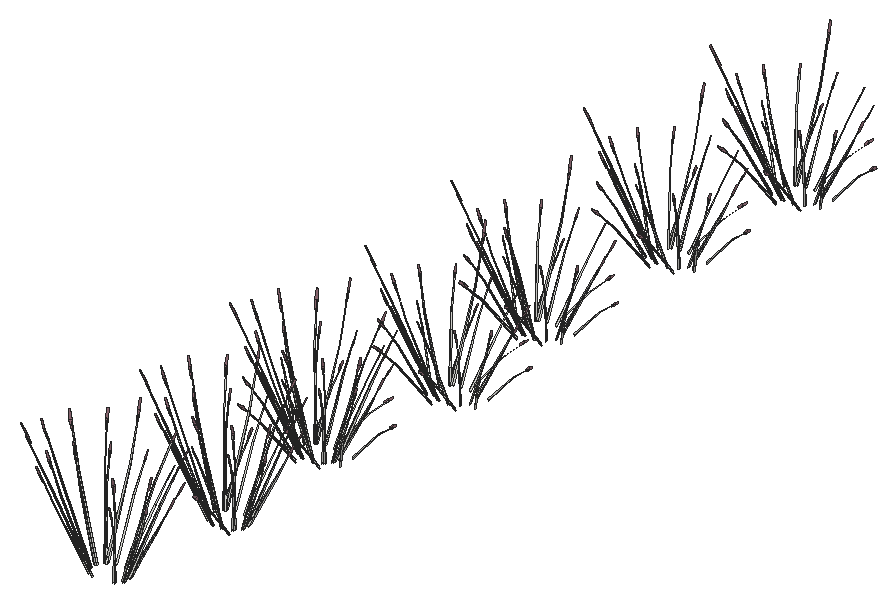
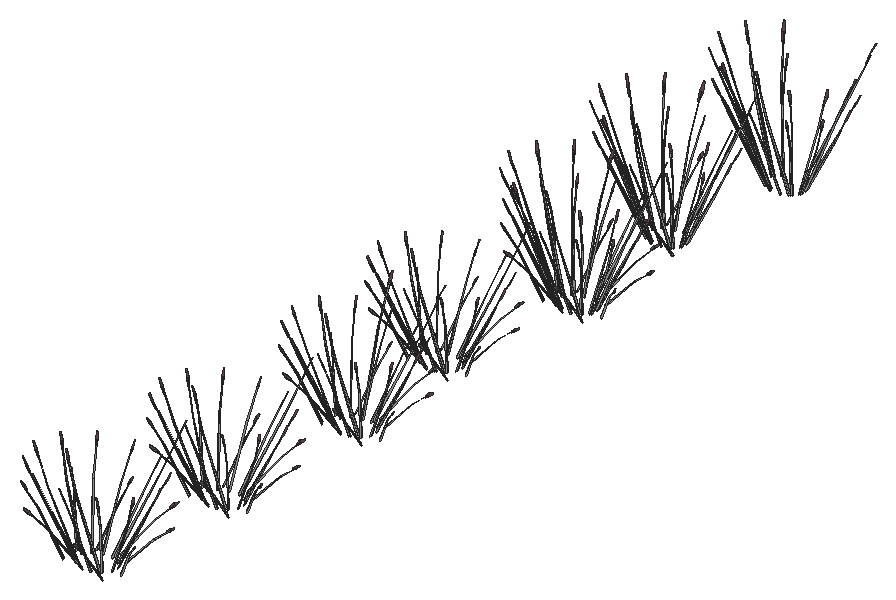
# SketchUp Ruby script. Lengths in inches.
U = 1.inch
M = Sketchup.active_model
def pt(a) = Geom::Point3d.new(a.map { |v| v * U })
def face(e, loops, mat)
  f = e.add_face(loops[0].map { |a| pt(a) })
  loops[1..].each { |l| e.add_face(l.map { |a| pt(a) }).erase! }
  f.material = f.back_material = mat if mat
  f
end
# faces: each face lists its corners as indices into pts; further lists are holes
def faces(e, pts, list, mat = nil) = list.each { |f| face(e, (f[0].is_a?(Array) ? f : [f]).map { |l| l.map { |i| pts[i] } }, mat) }
# xy, xz, yz: faces in a plane at the given z, y or x. An outline is a flat list of corners, or four numbers for a rectangle; further outlines are holes
def ring(l) = l.size == 4 ? [[l[0], l[1]], [l[2], l[1]], [l[2], l[3]], [l[0], l[3]]] : l.each_slice(2).to_a
def flat(e, list, mat, &to3) = list.each { |f| face(e, (f[0].is_a?(Array) ? f : [f]).map { |l| ring(l).map { |u, v| to3.(u, v) } }, mat) }
def xy(e, z, list, mat = nil) = flat(e, list, mat) { |x, y| [x, y, z] }
def xz(e, y, list, mat = nil) = flat(e, list, mat) { |x, z| [x, y, z] }
def yz(e, x, list, mat = nil) = flat(e, list, mat) { |y, z| [x, y, z] }
def lines(e, pts, list) = list.each { |a, b| e.add_line(pt(pts[a]), pt(pts[b])) }
# prism: a flat outline (further loops are holes) pulled along v
def prism(e, loops, v, mat = nil)
  f = face(e, loops, mat); d = Geom::Vector3d.new(v.map { |x| x * U })
  f.pushpull(f.normal.samedirection?(d) ? d.length : -d.length)
end
def box(e, o, s, mat = nil) = prism(e, [[o, [o[0] + s[0], o[1], o[2]], [o[0] + s[0], o[1] + s[1], o[2]], [o[0], o[1] + s[1], o[2]]]], [0, 0, s[2]], mat)
def at(x, y, z, deg = 0) = Geom::Transformation.translation(pt([x, y, z])) * Geom::Transformation.rotation(ORIGIN, Z_AXIS, deg.degrees)
def axes(o, x, y, z) = Geom::Transformation.new([*x, 0, *y, 0, *z, 0, *pt(o).to_a, 1])
def part(name) = M.definitions.add(name)
# library, detail: a bought-in or finely detailed component or shape, given as its bounding box
def library(name, o, s) = part(name).tap { |d| box(d.entities, o, s) }
def detail(e, o, s) = box(e.add_group.entities, o, s)
def put(e, d, t, mat = nil) = e.add_instance(d, t).tap { |i| i.material = mat if mat }
def group(e, t, mat = nil) = e.add_group.tap { |g| g.transformation = t; g.material = mat if mat }.entities
root = M.entities
M.materials.add("LightPink_Translucent").color = [144, 107, 117]
c1 = part("blade")
p = [[2.15,0.21,22],[0,0.17,0],[0.09,0.45,0],[2.18,0.31,22],[2.29,0.31,22],[0.38,0.45,0],
  [2.48,0.24,33],[2.49,0.24,33],[2.48,0.22,33]]
faces(c1.entities,p,[[0,1,2,3],[4,5,2,3],[6,3,4,7],[8,0,3,6]])
c2 = part("seeds")
p = [[0.3,-0.1,1.38],[-0.01,-0.03,1.59],[-0.01,-0.03,0.03],[0.14,-0.07,-0.07],[0.29,-0.03,3],[0.15,0.01,3.11]]
faces(c2.entities,p,[[0,1,2,3],[1,0,4,5]],"LightPink_Translucent")
c3 = part("blade with seeds")
put(c3.entities,c1,at(0,0,0))
put(c3.entities,c2,axes([2.4,0.25,30.99],[1.5799,-0.05474,1.17369],[-0.12525,1.92788,0.29478],[-0.07173,-0.02425,1.56792]))
put(root,c3,axes([46.34,429.16,46.73],[0.87265,0.70663,0.48003],[-0.92674,0.60943,0.3958],[0.16097,-0.33153,0.9933]))
put(root,c3,axes([41.07,428.13,47.43],[-0.81789,0.99285,-0.13619],[-1.18445,-0.572,-0.75594],[-0.41173,-0.28051,1.14864]))
put(root,c3,axes([46.66,429.23,46.73],[1.00708,0.04826,0.0643],[-0.02761,0.72867,0.50621],[0.10538,-0.27912,0.77189]))
put(root,c3,axes([38.21,429.49,46.73],[0.06171,-0.78753,0.0643],[0.9318,0.02159,0.50621],[-0.35694,-0.08241,0.77189]))
put(root,c3,axes([48.3125,431.27,46.73],[0.8413,0.43556,0.0643],[-0.48981,0.62025,0.50621],[0.26973,-0.20053,0.77189]))
put(root,c3,axes([48.08,431.09,46.73],[0.30393,0.95317,0.48003],[-1.19224,0.16542,0.3958],[0.35138,-0.22417,0.9933]))
put(root,c3,axes([36.85,431.89,46.73],[0.34623,-0.9443,0.48003],[1.13828,0.3229,0.3958],[-0.44763,0.05675,0.9933]))
put(root,c3,axes([36.77,431.64,46.73],[-0.4501,-0.70615,0.0643],[0.82077,-0.34564,0.50621],[-0.36181,0.0682,0.77189]))
put(root,c3,axes([48.4375,433.69,46.73],[0.4501,0.70615,0.0643],[-0.82077,0.34564,0.50621],[0.36181,-0.0682,0.77189]))
put(root,c3,axes([48.35,433.44,46.73],[-0.34623,0.9443,0.48003],[-1.13828,-0.3229,0.3958],[0.44763,-0.05675,0.9933]))
put(root,c3,axes([37.13,434.24,46.73],[-0.30393,-0.95317,0.48003],[1.19224,-0.16542,0.3958],[-0.35138,0.22417,0.9933]))
put(root,c3,axes([36.89,434.06,46.73],[-0.8413,-0.43556,0.0643],[0.48981,-0.62025,0.50621],[-0.26973,0.20053,0.77189]))
put(root,c3,axes([47,435.84,46.73],[-0.06171,0.78753,0.0643],[-0.9318,-0.02159,0.50621],[0.35694,0.08241,0.77189]))
put(root,c3,axes([47.09,435.58,46.73],[-0.90362,0.68241,0.48003],[-0.77932,-0.72471,0.3958],[0.42395,0.12588,0.9933]))
put(root,c3,axes([38.55,436.1,46.73],[-1.00708,-0.04826,0.0643],[0.02761,-0.72867,0.50621],[-0.10538,0.27912,0.77189]))
put(root,c3,axes([38.87,436.17,46.73],[-0.87265,-0.70663,0.48003],[0.92674,-0.60943,0.3958],[-0.16097,0.33153,0.9933]))
put(root,c3,axes([44.38,437.13,46.73],[-0.55698,0.6579,0.0643],[-0.79316,-0.38303,0.50621],[0.25643,0.21093,0.77189]))
put(root,c3,axes([44.62,436.95,46.73],[-1.21888,0.23767,0.48003],[-0.21154,-0.93233,0.3958],[0.28666,0.27478,0.9933]))
put(root,c3,axes([41.29,437.23,46.73],[-0.90301,0.35198,0.0643],[-0.44199,-0.64184,0.50621],[0.08721,0.28293,0.77189]))
put(root,c3,axes([38.77,435.76,47.4],[1.34686,0.05131,-0.13498],[-0.03681,0.97156,-0.74919],[-0.09356,0.37418,1.13838]))
put(root,c3,axes([53.75,466.55,46.71],[-0.12446,0.07911,1.77383],[-1.21937,-0.26689,-0.16761],[-0.04414,-0.34521,0.31391]))
put(root,c3,axes([49.95,467.43,46.73],[1.20755,0.27075,0.48003],[-0.41292,0.89013,0.3958],[-0.07257,-0.35005,0.9933]))
put(root,c3,axes([50.27,467.37,46.73],[0.90301,-0.35198,0.0643],[0.44199,0.64184,0.50621],[-0.08721,-0.28293,0.77189]))
put(root,c3,axes([47.18,467.46,46.73],[0.55698,-0.6579,0.0643],[0.79316,0.38303,0.50621],[-0.25643,-0.21093,0.77189]))
put(root,c3,axes([52.69,468.42,46.73],[0.87265,0.70663,0.48003],[-0.92674,0.60943,0.3958],[0.16097,-0.33153,0.9933]))
put(root,c3,axes([47.43,467.4,47.43],[-0.81789,0.99285,-0.13619],[-1.18445,-0.572,-0.75594],[-0.41173,-0.28051,1.14864]))
put(root,c3,axes([53.01,468.49,46.73],[1.00708,0.04826,0.0643],[-0.02761,0.72867,0.50621],[0.10538,-0.27912,0.77189]))
put(root,c3,axes([44.5625,468.76,46.73],[0.06171,-0.78753,0.0643],[0.9318,0.02159,0.50621],[-0.35694,-0.08241,0.77189]))
put(root,c3,axes([54.67,470.54,46.73],[0.8413,0.43556,0.0643],[-0.48981,0.62025,0.50621],[0.26973,-0.20053,0.77189]))
put(root,c3,axes([54.43,470.35,46.73],[0.30393,0.95317,0.48003],[-1.19224,0.16542,0.3958],[0.35138,-0.22417,0.9933]))
put(root,c3,axes([43.21,471.15,46.73],[0.34623,-0.9443,0.48003],[1.13828,0.3229,0.3958],[-0.44763,0.05675,0.9933]))
put(root,c3,axes([43.12,470.9,46.73],[-0.4501,-0.70615,0.0643],[0.82077,-0.34564,0.50621],[-0.36181,0.0682,0.77189]))
put(root,c3,axes([54.79,472.96,46.73],[0.4501,0.70615,0.0643],[-0.82077,0.34564,0.50621],[0.36181,-0.0682,0.77189]))
put(root,c3,axes([54.71,472.71,46.73],[-0.34623,0.9443,0.48003],[-1.13828,-0.3229,0.3958],[0.44763,-0.05675,0.9933]))
put(root,c3,axes([43.48,473.51,46.73],[-0.30393,-0.95317,0.48003],[1.19224,-0.16542,0.3958],[-0.35138,0.22417,0.9933]))
put(root,c3,axes([43.25,473.32,46.73],[-0.8413,-0.43556,0.0643],[0.48981,-0.62025,0.50621],[-0.26973,0.20053,0.77189]))
put(root,c3,axes([53.36,475.1,46.73],[-0.06171,0.78753,0.0643],[-0.9318,-0.02159,0.50621],[0.35694,0.08241,0.77189]))
put(root,c3,axes([53.44,474.85,46.73],[-0.90362,0.68241,0.48003],[-0.77932,-0.72471,0.3958],[0.42395,0.12588,0.9933]))
put(root,c3,axes([44.9,475.37,46.73],[-1.00708,-0.04826,0.0643],[0.02761,-0.72867,0.50621],[-0.10538,0.27912,0.77189]))
put(root,c3,axes([45.23,475.4375,46.73],[-0.87265,-0.70663,0.48003],[0.92674,-0.60943,0.3958],[-0.16097,0.33153,0.9933]))
put(root,c3,axes([50.74,476.4,46.73],[-0.55698,0.6579,0.0643],[-0.79316,-0.38303,0.50621],[0.25643,0.21093,0.77189]))
put(root,c3,axes([50.97,476.21,46.73],[-1.21888,0.23767,0.48003],[-0.21154,-0.93233,0.3958],[0.28666,0.27478,0.9933]))
put(root,c3,axes([47.65,476.49,46.73],[-0.90301,0.35198,0.0643],[-0.44199,-0.64184,0.50621],[0.08721,0.28293,0.77189]))
put(root,c3,axes([45.13,475.02,47.4],[1.34686,0.05131,-0.13498],[-0.03681,0.97156,-0.74919],[-0.09356,0.37418,1.13838]))
put(root,c3,axes([42.27,477.59,46.71],[0.13903,-0.06253,1.77383],[1.14912,0.41591,-0.16761],[-0.027,0.34629,0.31391]))
put(root,c3,axes([50.13,506.81,46.71],[-0.12446,0.07911,1.77383],[-1.21937,-0.26689,-0.16761],[-0.04414,-0.34521,0.31391]))
put(root,c3,axes([43.5,505.29,46.71],[-0.02286,0.12414,1.77383],[-1.12758,0.45052,-0.16761],[-0.33182,-0.23029,0.31391]))
put(root,c3,axes([46.34,507.69,46.73],[1.20755,0.27075,0.48003],[-0.41292,0.89013,0.3958],[-0.07257,-0.35005,0.9933]))
put(root,c3,axes([46.66,507.625,46.73],[0.90301,-0.35198,0.0643],[0.44199,0.64184,0.50621],[-0.08721,-0.28293,0.77189]))
put(root,c3,axes([43.5625,507.72,46.73],[0.55698,-0.6579,0.0643],[0.79316,0.38303,0.50621],[-0.25643,-0.21093,0.77189]))
put(root,c3,axes([49.08,508.68,46.73],[0.87265,0.70663,0.48003],[-0.92674,0.60943,0.3958],[0.16097,-0.33153,0.9933]))
put(root,c3,axes([43.8125,507.65,47.43],[-0.81789,0.99285,-0.13619],[-1.18445,-0.572,-0.75594],[-0.41173,-0.28051,1.14864]))
put(root,c3,axes([49.4,508.75,46.73],[1.00708,0.04826,0.0643],[-0.02761,0.72867,0.50621],[0.10538,-0.27912,0.77189]))
put(root,c3,axes([53.43,510.76,46.71],[-0.16006,-0.00787,1.77383],[-0.66468,-0.8428,-0.16761],[0.26693,-0.27711,0.31391]))
put(root,c3,axes([40.95,509.02,46.73],[0.06171,-0.78753,0.0643],[0.9318,0.02159,0.50621],[-0.35694,-0.08241,0.77189]))
put(root,c3,axes([51.05,510.8,46.73],[0.8413,0.43556,0.0643],[-0.48981,0.62025,0.50621],[0.26973,-0.20053,0.77189]))
put(root,c3,axes([50.82,510.61,46.73],[0.30393,0.95317,0.48003],[-1.19224,0.16542,0.3958],[0.35138,-0.22417,0.9933]))
put(root,c3,axes([39.66,507.99,46.71],[0.09085,0.10335,1.77383],[-0.43798,0.92907,-0.16761],[-0.44357,0.00672,0.31391]))
put(root,c3,axes([39.59,511.41,46.73],[0.34623,-0.9443,0.48003],[1.13828,0.3229,0.3958],[-0.44763,0.05675,0.9933]))
put(root,c3,axes([39.51,511.16,46.73],[-0.4501,-0.70615,0.0643],[0.82077,-0.34564,0.50621],[-0.36181,0.0682,0.77189]))
put(root,c3,axes([51.18,513.21,46.73],[0.4501,0.70615,0.0643],[-0.82077,0.34564,0.50621],[0.36181,-0.0682,0.77189]))
put(root,c3,axes([51.09,512.96,46.73],[-0.34623,0.9443,0.48003],[-1.13828,-0.3229,0.3958],[0.44763,-0.05675,0.9933]))
put(root,c3,axes([53.14,516.02,46.71],[-0.11081,-0.09067,1.77383],[0.2424,-0.97188,-0.16761],[0.43649,-0.06209,0.31391]))
put(root,c3,axes([39.87,513.76,46.73],[-0.30393,-0.95317,0.48003],[1.19224,-0.16542,0.3958],[-0.35138,0.22417,0.9933]))
put(root,c3,axes([39.63,513.58,46.73],[-0.8413,-0.43556,0.0643],[0.48981,-0.62025,0.50621],[-0.26973,0.20053,0.77189]))
put(root,c3,axes([36.49,513.07,46.71],[0.1564,0.02778,1.77383],[0.48382,0.91506,-0.16761],[-0.32016,0.24017,0.31391]))
put(root,c3,axes([49.74,515.36,46.73],[-0.06171,0.78753,0.0643],[-0.9318,-0.02159,0.50621],[0.35694,0.08241,0.77189]))
put(root,c3,axes([49.83,515.11,46.73],[-0.90362,0.68241,0.48003],[-0.77932,-0.72471,0.3958],[0.42395,0.12588,0.9933]))
put(root,c3,axes([45.9,517.07,46.71],[0.00363,-0.12539,1.77383],[1.0502,-0.55319,-0.16761],[0.36479,0.19745,0.31391]))
put(root,c3,axes([41.29,515.63,46.73],[-1.00708,-0.04826,0.0643],[0.02761,-0.72867,0.50621],[-0.10538,0.27912,0.77189]))
put(root,c3,axes([41.61,515.69,46.73],[-0.87265,-0.70663,0.48003],[0.92674,-0.60943,0.3958],[-0.16097,0.33153,0.9933]))
put(root,c3,axes([47.125,516.65,46.73],[-0.55698,0.6579,0.0643],[-0.79316,-0.38303,0.50621],[0.25643,0.21093,0.77189]))
put(root,c3,axes([47.36,516.47,46.73],[-1.21888,0.23767,0.48003],[-0.21154,-0.93233,0.3958],[0.28666,0.27478,0.9933]))
put(root,c3,axes([44.03,516.75,46.73],[-0.90301,0.35198,0.0643],[-0.44199,-0.64184,0.50621],[0.08721,0.28293,0.77189]))
put(root,c3,axes([41.51,515.28,47.4],[1.34686,0.05131,-0.13498],[-0.03681,0.97156,-0.74919],[-0.09356,0.37418,1.13838]))
put(root,c3,axes([38.65,517.85,46.71],[0.13903,-0.06253,1.77383],[1.14912,0.41591,-0.16761],[-0.027,0.34629,0.31391]))
put(root,c3,axes([58.1,550.49,46.71],[-0.12446,0.07911,1.77383],[-1.21937,-0.26689,-0.16761],[-0.04414,-0.34521,0.31391]))
put(root,c3,axes([51.46,548.97,46.71],[-0.02286,0.12414,1.77383],[-1.12758,0.45052,-0.16761],[-0.33182,-0.23029,0.31391]))
put(root,c3,axes([54.625,551.3,46.73],[0.90301,-0.35198,0.0643],[0.44199,0.64184,0.50621],[-0.08721,-0.28293,0.77189]))
put(root,c3,axes([51.53,551.4,46.73],[0.55698,-0.6579,0.0643],[0.79316,0.38303,0.50621],[-0.25643,-0.21093,0.77189]))
put(root,c3,axes([51.78,551.33,47.43],[-0.81789,0.99285,-0.13619],[-1.18445,-0.572,-0.75594],[-0.41173,-0.28051,1.14864]))
put(root,c3,axes([57.37,552.42,46.73],[1.00708,0.04826,0.0643],[-0.02761,0.72867,0.50621],[0.10538,-0.27912,0.77189]))
put(root,c3,axes([61.4,554.43,46.71],[-0.16006,-0.00787,1.77383],[-0.66468,-0.8428,-0.16761],[0.26693,-0.27711,0.31391]))
put(root,c3,axes([48.91,552.69,46.73],[0.06171,-0.78753,0.0643],[0.9318,0.02159,0.50621],[-0.35694,-0.08241,0.77189]))
put(root,c3,axes([59.02,554.47,46.73],[0.8413,0.43556,0.0643],[-0.48981,0.62025,0.50621],[0.26973,-0.20053,0.77189]))
put(root,c3,axes([47.63,551.66,46.71],[0.09085,0.10335,1.77383],[-0.43798,0.92907,-0.16761],[-0.44357,0.00672,0.31391]))
put(root,c3,axes([47.48,554.84,46.73],[-0.4501,-0.70615,0.0643],[0.82077,-0.34564,0.50621],[-0.36181,0.0682,0.77189]))
put(root,c3,axes([59.15,556.89,46.73],[0.4501,0.70615,0.0643],[-0.82077,0.34564,0.50621],[0.36181,-0.0682,0.77189]))
put(root,c3,axes([61.11,559.7,46.71],[-0.11081,-0.09067,1.77383],[0.2424,-0.97188,-0.16761],[0.43649,-0.06209,0.31391]))
put(root,c3,axes([47.6,557.26,46.73],[-0.8413,-0.43556,0.0643],[0.48981,-0.62025,0.50621],[-0.26973,0.20053,0.77189]))
put(root,c3,axes([44.46,556.75,46.71],[0.1564,0.02778,1.77383],[0.48382,0.91506,-0.16761],[-0.32016,0.24017,0.31391]))
put(root,c3,axes([57.71,559.03,46.73],[-0.06171,0.78753,0.0643],[-0.9318,-0.02159,0.50621],[0.35694,0.08241,0.77189]))
put(root,c3,axes([53.87,560.74,46.71],[0.00363,-0.12539,1.77383],[1.0502,-0.55319,-0.16761],[0.36479,0.19745,0.31391]))
put(root,c3,axes([49.26,559.3,46.73],[-1.00708,-0.04826,0.0643],[0.02761,-0.72867,0.50621],[-0.10538,0.27912,0.77189]))
put(root,c3,axes([55.09,560.33,46.73],[-0.55698,0.6579,0.0643],[-0.79316,-0.38303,0.50621],[0.25643,0.21093,0.77189]))
put(root,c3,axes([52,560.43,46.73],[-0.90301,0.35198,0.0643],[-0.44199,-0.64184,0.50621],[0.08721,0.28293,0.77189]))
put(root,c3,axes([49.48,558.96,47.4],[1.34686,0.05131,-0.13498],[-0.03681,0.97156,-0.74919],[-0.09356,0.37418,1.13838]))
put(root,c3,axes([46.62,561.52,46.71],[0.13903,-0.06253,1.77383],[1.14912,0.41591,-0.16761],[-0.027,0.34629,0.31391]))
put(root,c3,axes([54.27,589.3125,46.71],[-0.12446,0.07911,1.77383],[-1.21937,-0.26689,-0.16761],[-0.04414,-0.34521,0.31391]))
put(root,c3,axes([47.63,587.79,46.71],[-0.02286,0.12414,1.77383],[-1.12758,0.45052,-0.16761],[-0.33182,-0.23029,0.31391]))
put(root,c3,axes([50.47,590.19,46.73],[1.20755,0.27075,0.48003],[-0.41292,0.89013,0.3958],[-0.07257,-0.35005,0.9933]))
put(root,c3,axes([50.79,590.125,46.73],[0.90301,-0.35198,0.0643],[0.44199,0.64184,0.50621],[-0.08721,-0.28293,0.77189]))
put(root,c3,axes([47.7,590.22,46.73],[0.55698,-0.6579,0.0643],[0.79316,0.38303,0.50621],[-0.25643,-0.21093,0.77189]))
put(root,c3,axes([47.95,590.15,47.43],[-0.81789,0.99285,-0.13619],[-1.18445,-0.572,-0.75594],[-0.41173,-0.28051,1.14864]))
put(root,c3,axes([53.54,591.25,46.73],[1.00708,0.04826,0.0643],[-0.02761,0.72867,0.50621],[0.10538,-0.27912,0.77189]))
put(root,c3,axes([57.57,593.26,46.71],[-0.16006,-0.00787,1.77383],[-0.66468,-0.8428,-0.16761],[0.26693,-0.27711,0.31391]))
put(root,c3,axes([45.08,591.52,46.73],[0.06171,-0.78753,0.0643],[0.9318,0.02159,0.50621],[-0.35694,-0.08241,0.77189]))
put(root,c3,axes([55.19,593.3,46.73],[0.8413,0.43556,0.0643],[-0.48981,0.62025,0.50621],[0.26973,-0.20053,0.77189]))
put(root,c3,axes([43.8,590.49,46.71],[0.09085,0.10335,1.77383],[-0.43798,0.92907,-0.16761],[-0.44357,0.00672,0.31391]))
put(root,c3,axes([43.65,593.66,46.73],[-0.4501,-0.70615,0.0643],[0.82077,-0.34564,0.50621],[-0.36181,0.0682,0.77189]))
put(root,c3,axes([55.32,595.72,46.73],[0.4501,0.70615,0.0643],[-0.82077,0.34564,0.50621],[0.36181,-0.0682,0.77189]))
put(root,c3,axes([57.28,598.52,46.71],[-0.11081,-0.09067,1.77383],[0.2424,-0.97188,-0.16761],[0.43649,-0.06209,0.31391]))
put(root,c3,axes([43.77,596.08,46.73],[-0.8413,-0.43556,0.0643],[0.48981,-0.62025,0.50621],[-0.26973,0.20053,0.77189]))
put(root,c3,axes([40.63,595.57,46.71],[0.1564,0.02778,1.77383],[0.48382,0.91506,-0.16761],[-0.32016,0.24017,0.31391]))
put(root,c3,axes([53.88,597.86,46.73],[-0.06171,0.78753,0.0643],[-0.9318,-0.02159,0.50621],[0.35694,0.08241,0.77189]))
put(root,c3,axes([50.04,599.57,46.71],[0.00363,-0.12539,1.77383],[1.0502,-0.55319,-0.16761],[0.36479,0.19745,0.31391]))
put(root,c3,axes([45.43,598.13,46.73],[-1.00708,-0.04826,0.0643],[0.02761,-0.72867,0.50621],[-0.10538,0.27912,0.77189]))
put(root,c3,axes([51.26,599.15,46.73],[-0.55698,0.6579,0.0643],[-0.79316,-0.38303,0.50621],[0.25643,0.21093,0.77189]))
put(root,c3,axes([48.17,599.25,46.73],[-0.90301,0.35198,0.0643],[-0.44199,-0.64184,0.50621],[0.08721,0.28293,0.77189]))
put(root,c3,axes([45.65,597.78,47.4],[1.34686,0.05131,-0.13498],[-0.03681,0.97156,-0.74919],[-0.09356,0.37418,1.13838]))
put(root,c3,axes([42.79,600.35,46.71],[0.13903,-0.06253,1.77383],[1.14912,0.41591,-0.16761],[-0.027,0.34629,0.31391]))
put(root,c3,axes([57.0625,638.32,46.71],[-0.12446,0.07911,1.77383],[-1.21937,-0.26689,-0.16761],[-0.04414,-0.34521,0.31391]))
put(root,c3,axes([50.43,636.8,46.71],[-0.02286,0.12414,1.77383],[-1.12758,0.45052,-0.16761],[-0.33182,-0.23029,0.31391]))
put(root,c3,axes([53.59,639.14,46.73],[0.90301,-0.35198,0.0643],[0.44199,0.64184,0.50621],[-0.08721,-0.28293,0.77189]))
put(root,c3,axes([50.49,639.23,46.73],[0.55698,-0.6579,0.0643],[0.79316,0.38303,0.50621],[-0.25643,-0.21093,0.77189]))
put(root,c3,axes([50.74,639.16,47.43],[-0.81789,0.99285,-0.13619],[-1.18445,-0.572,-0.75594],[-0.41173,-0.28051,1.14864]))
put(root,c3,axes([56.33,640.26,46.73],[1.00708,0.04826,0.0643],[-0.02761,0.72867,0.50621],[0.10538,-0.27912,0.77189]))
put(root,c3,axes([60.36,642.27,46.71],[-0.16006,-0.00787,1.77383],[-0.66468,-0.8428,-0.16761],[0.26693,-0.27711,0.31391]))
put(root,c3,axes([47.875,640.53,46.73],[0.06171,-0.78753,0.0643],[0.9318,0.02159,0.50621],[-0.35694,-0.08241,0.77189]))
put(root,c3,axes([57.98,642.31,46.73],[0.8413,0.43556,0.0643],[-0.48981,0.62025,0.50621],[0.26973,-0.20053,0.77189]))
put(root,c3,axes([46.59,639.5,46.71],[0.09085,0.10335,1.77383],[-0.43798,0.92907,-0.16761],[-0.44357,0.00672,0.31391]))
put(root,c3,axes([46.4375,642.67,46.73],[-0.4501,-0.70615,0.0643],[0.82077,-0.34564,0.50621],[-0.36181,0.0682,0.77189]))
put(root,c3,axes([58.11,644.72,46.73],[0.4501,0.70615,0.0643],[-0.82077,0.34564,0.50621],[0.36181,-0.0682,0.77189]))
put(root,c3,axes([60.07,647.53,46.71],[-0.11081,-0.09067,1.77383],[0.2424,-0.97188,-0.16761],[0.43649,-0.06209,0.31391]))
put(root,c3,axes([46.5625,645.09,46.73],[-0.8413,-0.43556,0.0643],[0.48981,-0.62025,0.50621],[-0.26973,0.20053,0.77189]))
put(root,c3,axes([43.42,644.58,46.71],[0.1564,0.02778,1.77383],[0.48382,0.91506,-0.16761],[-0.32016,0.24017,0.31391]))
put(root,c3,axes([56.67,646.87,46.73],[-0.06171,0.78753,0.0643],[-0.9318,-0.02159,0.50621],[0.35694,0.08241,0.77189]))
put(root,c3,axes([52.83,648.58,46.71],[0.00363,-0.12539,1.77383],[1.0502,-0.55319,-0.16761],[0.36479,0.19745,0.31391]))
put(root,c3,axes([48.22,647.14,46.73],[-1.00708,-0.04826,0.0643],[0.02761,-0.72867,0.50621],[-0.10538,0.27912,0.77189]))
put(root,c3,axes([54.05,648.16,46.73],[-0.55698,0.6579,0.0643],[-0.79316,-0.38303,0.50621],[0.25643,0.21093,0.77189]))
put(root,c3,axes([50.96,648.26,46.73],[-0.90301,0.35198,0.0643],[-0.44199,-0.64184,0.50621],[0.08721,0.28293,0.77189]))
put(root,c3,axes([48.44,646.79,47.4],[1.34686,0.05131,-0.13498],[-0.03681,0.97156,-0.74919],[-0.09356,0.37418,1.13838]))
put(root,c3,axes([45.58,649.36,46.71],[0.13903,-0.06253,1.77383],[1.14912,0.41591,-0.16761],[-0.027,0.34629,0.31391]))
put(root,c3,axes([61.6,682.65,46.71],[-0.12446,0.07911,1.77383],[-1.21937,-0.26689,-0.16761],[-0.04414,-0.34521,0.31391]))
put(root,c3,axes([54.97,681.13,46.71],[-0.02286,0.12414,1.77383],[-1.12758,0.45052,-0.16761],[-0.33182,-0.23029,0.31391]))
put(root,c3,axes([58.125,683.46,46.73],[0.90301,-0.35198,0.0643],[0.44199,0.64184,0.50621],[-0.08721,-0.28293,0.77189]))
put(root,c3,axes([55.03,683.5625,46.73],[0.55698,-0.6579,0.0643],[0.79316,0.38303,0.50621],[-0.25643,-0.21093,0.77189]))
put(root,c3,axes([55.28,683.49,47.43],[-0.81789,0.99285,-0.13619],[-1.18445,-0.572,-0.75594],[-0.41173,-0.28051,1.14864]))
put(root,c3,axes([60.87,684.59,46.73],[1.00708,0.04826,0.0643],[-0.02761,0.72867,0.50621],[0.10538,-0.27912,0.77189]))
put(root,c3,axes([64.9,686.6,46.71],[-0.16006,-0.00787,1.77383],[-0.66468,-0.8428,-0.16761],[0.26693,-0.27711,0.31391]))
put(root,c3,axes([52.42,684.86,46.73],[0.06171,-0.78753,0.0643],[0.9318,0.02159,0.50621],[-0.35694,-0.08241,0.77189]))
put(root,c3,axes([62.52,686.63,46.73],[0.8413,0.43556,0.0643],[-0.48981,0.62025,0.50621],[0.26973,-0.20053,0.77189]))
put(root,c3,axes([51.13,683.83,46.71],[0.09085,0.10335,1.77383],[-0.43798,0.92907,-0.16761],[-0.44357,0.00672,0.31391]))
put(root,c3,axes([50.98,687,46.73],[-0.4501,-0.70615,0.0643],[0.82077,-0.34564,0.50621],[-0.36181,0.0682,0.77189]))
put(root,c3,axes([62.65,689.05,46.73],[0.4501,0.70615,0.0643],[-0.82077,0.34564,0.50621],[0.36181,-0.0682,0.77189]))
put(root,c3,axes([64.61,691.86,46.71],[-0.11081,-0.09067,1.77383],[0.2424,-0.97188,-0.16761],[0.43649,-0.06209,0.31391]))
put(root,c3,axes([51.1,689.42,46.73],[-0.8413,-0.43556,0.0643],[0.48981,-0.62025,0.50621],[-0.26973,0.20053,0.77189]))
put(root,c3,axes([47.96,688.91,46.71],[0.1564,0.02778,1.77383],[0.48382,0.91506,-0.16761],[-0.32016,0.24017,0.31391]))
put(root,c3,axes([61.21,691.2,46.73],[-0.06171,0.78753,0.0643],[-0.9318,-0.02159,0.50621],[0.35694,0.08241,0.77189]))
put(root,c3,axes([57.37,692.9,46.71],[0.00363,-0.12539,1.77383],[1.0502,-0.55319,-0.16761],[0.36479,0.19745,0.31391]))
put(root,c3,axes([52.76,691.47,46.73],[-1.00708,-0.04826,0.0643],[0.02761,-0.72867,0.50621],[-0.10538,0.27912,0.77189]))
put(root,c3,axes([58.59,692.49,46.73],[-0.55698,0.6579,0.0643],[-0.79316,-0.38303,0.50621],[0.25643,0.21093,0.77189]))
put(root,c3,axes([55.5,692.59,46.73],[-0.90301,0.35198,0.0643],[-0.44199,-0.64184,0.50621],[0.08721,0.28293,0.77189]))
put(root,c3,axes([52.98,691.12,47.4],[1.34686,0.05131,-0.13498],[-0.03681,0.97156,-0.74919],[-0.09356,0.37418,1.13838]))
put(root,c3,axes([50.12,693.6875,46.71],[0.13903,-0.06253,1.77383],[1.14912,0.41591,-0.16761],[-0.027,0.34629,0.31391]))
